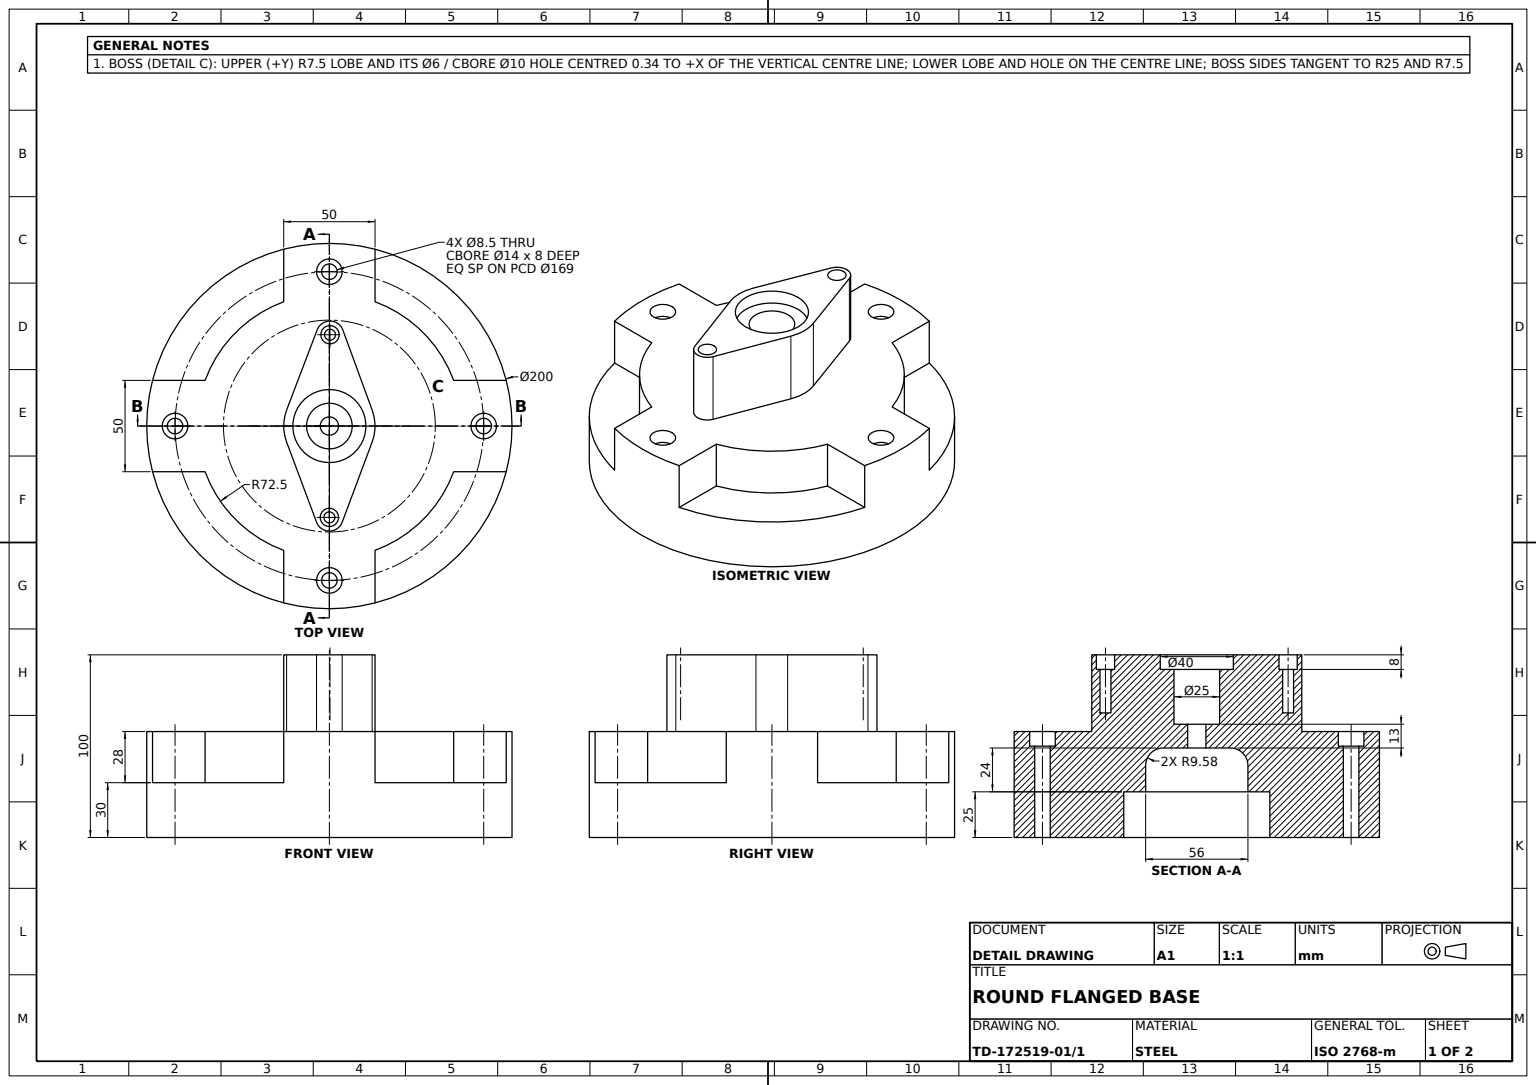
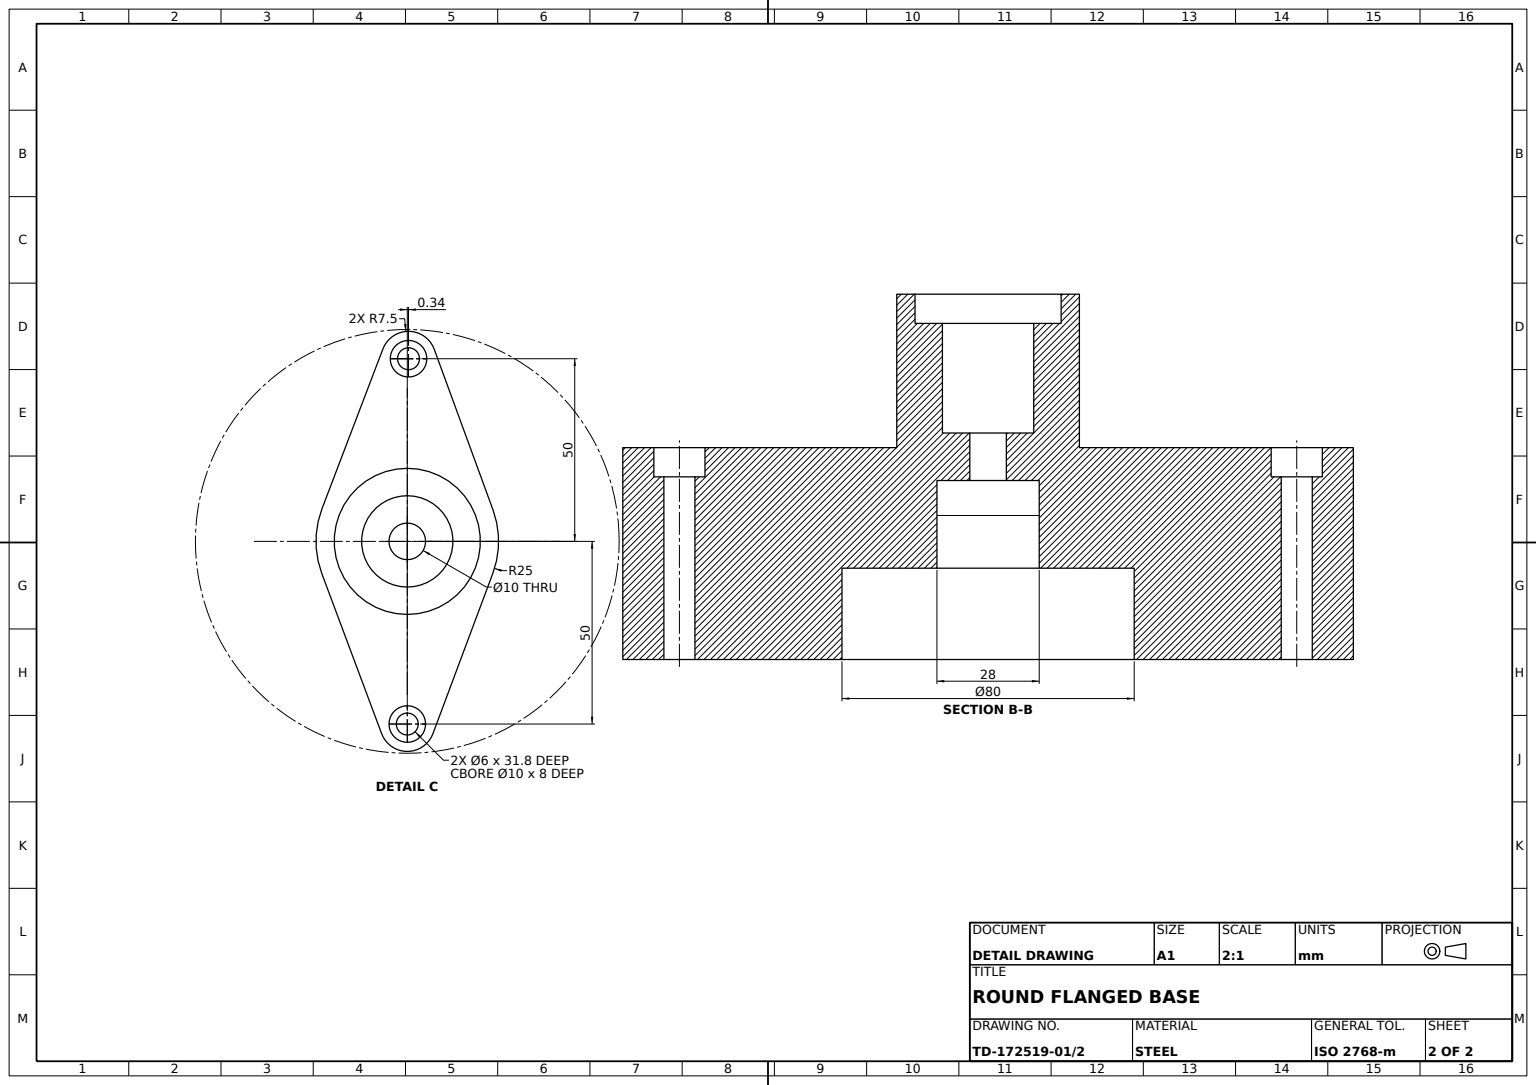
solid
v1 (0,68.2,53)
v2 (0,68.2,47)
e1 v1 v2 CIRCLE(AX(P(0,68.2,50),D(0,1,0),D(0,0,1)),3)
e2 v2 v1 CIRCLE(AX(P(0,68.2,50),D(0,1,0),D(0,0,1)),3)
face PLANE(AX(P(0,68.2,50),D(0,1,0),D(0,0,1))) [e1 e2]
v3 (0,58,-91.5)
v4 (0,58,-77.5)
e3 v3 v4 CIRCLE(AX(P(0,58,-84.5),D(0,1,0),D(0,0,1)),7)
e4 v4 v3 CIRCLE(AX(P(0,58,-84.5),D(0,1,0),D(0,0,1)),7)
v5 (25,58,68.053288)
v6 (68.053288,58,25)
e5 v5 v6 CIRCLE(AX(P(0,58,0),D(0,1,0),D(0,0,1)),72.5)
v7 (96.824584,58,25)
e6 v6 v7 LINE
v8 (96.824584,58,-25)
e7 v7 v8 CIRCLE(AX(P(0,58,0),D(0,1,0),D(0,0,1)),100)
v9 (68.053288,58,-25)
e8 v8 v9 LINE
v10 (25,58,-68.053288)
e9 v9 v10 CIRCLE(AX(P(0,58,0),D(0,1,0),D(0,0,1)),72.5)
v11 (25,58,-96.824584)
e10 v10 v11 LINE
v12 (0,58,-100)
e11 v11 v12 CIRCLE(AX(P(0,58,0),D(0,1,0),D(0,0,1)),100)
v13 (-25,58,-96.824584)
e12 v12 v13 CIRCLE(AX(P(0,58,0),D(0,1,0),D(0,0,1)),100)
v14 (-25,58,-68.053288)
e13 v13 v14 LINE
v15 (-68.053288,58,-25)
e14 v14 v15 CIRCLE(AX(P(0,58,0),D(0,1,0),D(0,0,1)),72.5)
v16 (-96.824584,58,-25)
e15 v15 v16 LINE
v17 (-96.824584,58,25)
e16 v16 v17 CIRCLE(AX(P(0,58,0),D(0,1,0),D(0,0,1)),100)
v18 (-68.053288,58,25)
e17 v17 v18 LINE
v19 (-25,58,68.053288)
e18 v18 v19 CIRCLE(AX(P(0,58,0),D(0,1,0),D(0,0,1)),72.5)
v20 (-25,58,96.824584)
e19 v19 v20 LINE
v21 (0,58,100)
e20 v20 v21 CIRCLE(AX(P(0,58,0),D(0,1,0),D(0,0,1)),100)
v22 (25,58,96.824584)
e21 v21 v22 CIRCLE(AX(P(0,58,0),D(0,1,0),D(0,0,1)),100)
e22 v22 v5 LINE
v23 (84.5,58,-7)
v24 (84.5,58,7)
e23 v23 v24 CIRCLE(AX(P(84.5,58,0),D(0,1,0),D(0,0,1)),7)
e24 v24 v23 CIRCLE(AX(P(84.5,58,0),D(0,1,0),D(0,0,1)),7)
v25 (0,58,77.5)
v26 (0,58,91.5)
e25 v25 v26 CIRCLE(AX(P(0,58,84.5),D(0,1,0),D(0,0,1)),7)
e26 v26 v25 CIRCLE(AX(P(0,58,84.5),D(0,1,0),D(0,0,1)),7)
v27 (7.025623,58,52.625)
v28 (23.418742,58,8.75)
e27 v27 v28 LINE
v29 (-7.025623,58,52.625)
e28 v29 v27 CIRCLE(AX(P(0,58,50),D(0,1,0),D(0,0,1)),7.5)
v30 (-23.418742,58,8.75)
e29 v30 v29 LINE
v31 (-23.359174,58,-8.907806)
e30 v31 v30 CIRCLE(AX(P(0,58,0),D(0,1,0),D(0,0,1)),25)
v32 (-6.670405,58,-52.671204)
e31 v32 v31 LINE
v33 (0.337347,58,-57.498862)
e32 v33 v32 CIRCLE(AX(P(0.337347,58,-49.998862),D(0,1,0),D(0,0,1)),7.5)
v34 (7.380521,58,-52.576401)
e33 v34 v33 CIRCLE(AX(P(0.337347,58,-49.998862),D(0,1,0),D(0,0,1)),7.5)
v35 (23.477245,58,-8.591796)
e34 v35 v34 LINE
e35 v28 v35 CIRCLE(AX(P(0,58,0),D(0,1,0),D(0,0,1)),25)
v36 (-84.5,58,7)
v37 (-84.5,58,-7)
e36 v36 v37 CIRCLE(AX(P(-84.5,58,0),D(0,1,0),D(0,0,1)),7)
e37 v37 v36 CIRCLE(AX(P(-84.5,58,0),D(0,1,0),D(0,0,1)),7)
face PLANE(AX(P(0,58,0),D(0,1,0),D(0,0,1))) [-e3 -e4] [e5 e6 e7 e8 e9 e10 e11 e12 e13 e14 e15 e16 e17 e18 e19 e20 e21 e22] [-e23 -e24] [-e25 -e26] [-e27 -e28 -e29 -e30 -e31 -e32 -e33 -e34 -e35] [-e36 -e37]
v38 (23.477245,100,-8.591796)
e38 v38 v35 LINE
v39 (23.418742,100,8.75)
e39 v39 v38 CIRCLE(AX(P(0,100,0),D(0,1,0),D(0,0,1)),25)
e40 v39 v28 LINE
face CYL(AX(P(0,100,0),D(0,-1,0),D(0,0,-1)),25) [-e38 -e39 e40 e35]
v40 (0,0,80.25)
v41 (0,0,88.75)
e41 v40 v41 CIRCLE(AX(P(0,0,84.5),D(0,1,0),D(0,0,1)),4.25)
e42 v41 v40 CIRCLE(AX(P(0,0,84.5),D(0,1,0),D(0,0,1)),4.25)
v42 (0,0,-80.25)
v43 (0,0,-88.75)
e43 v42 v43 CIRCLE(AX(P(0,0,-84.5),D(0,1,0),D(0,0,1)),4.25)
e44 v43 v42 CIRCLE(AX(P(0,0,-84.5),D(0,1,0),D(0,0,1)),4.25)
v44 (0,0,-100)
v45 (0,0,100)
e45 v44 v45 CIRCLE(AX(P(0,0,0),D(0,1,0),D(0,0,1)),100)
e46 v45 v44 CIRCLE(AX(P(0,0,0),D(0,1,0),D(0,0,1)),100)
v46 (-84.5,0,4.25)
v47 (-84.5,0,-4.25)
e47 v46 v47 CIRCLE(AX(P(-84.5,0,0),D(0,1,0),D(0,0,1)),4.25)
e48 v47 v46 CIRCLE(AX(P(-84.5,0,0),D(0,1,0),D(0,0,1)),4.25)
v48 (84.5,0,4.25)
v49 (84.5,0,-4.25)
e49 v48 v49 CIRCLE(AX(P(84.5,0,0),D(0,1,0),D(0,0,1)),4.25)
e50 v49 v48 CIRCLE(AX(P(84.5,0,0),D(0,1,0),D(0,0,1)),4.25)
v50 (0,0,-40)
v51 (0,0,40)
e51 v50 v51 CIRCLE(AX(P(0,0,0),D(0,-1,0),D(0,0,-1)),40)
e52 v51 v50 CIRCLE(AX(P(0,0,0),D(0,-1,0),D(0,0,-1)),40)
face PLANE(AX(P(0,0,0),D(0,1,0),D(0,0,1))) rev [e41 e42] [e43 e44] [-e45 -e46] [e47 e48] [e49 e50] [-e51 -e52]
v52 (-84.5,50,7)
e53 v52 v36 LINE
v53 (-84.5,50,-7)
e54 v53 v37 LINE
e55 v52 v53 CIRCLE(AX(P(-84.5,50,0),D(0,1,0),D(0,0,1)),7)
face CYL(AX(P(-84.5,50,0),D(0,1,0),D(0,0,1)),7) rev [e53 e36 -e54 -e55]
v54 (0.337347,100,-44.998862)
v55 (0.337347,100,-54.998862)
e56 v54 v55 CIRCLE(AX(P(0.337347,100,-49.998862),D(0,1,0),D(0,0,1)),5)
v56 (0.337347,92,-54.998862)
e57 v56 v55 LINE
v57 (0.337347,92,-44.998862)
e58 v57 v56 CIRCLE(AX(P(0.337347,92,-49.998862),D(0,1,0),D(0,0,1)),5)
e59 v57 v54 LINE
face CYL(AX(P(0.337347,92,-49.998862),D(0,1,0),D(0,0,1)),5) rev [e56 -e57 -e58 e59]
v58 (0.337347,68.2,-52.998862)
v59 (0.337347,68.2,-46.998862)
e60 v58 v59 CIRCLE(AX(P(0.337347,68.2,-49.998862),D(0,1,0),D(0,0,1)),3)
e61 v59 v58 CIRCLE(AX(P(0.337347,68.2,-49.998862),D(0,1,0),D(0,0,1)),3)
face PLANE(AX(P(0.337347,68.2,-49.998862),D(0,1,0),D(0,0,1))) [e60 e61]
v60 (-96.824584,30,25)
v61 (-25,30,96.824584)
e62 v60 v61 CIRCLE(AX(P(0,30,0),D(0,1,0),D(0,0,1)),100)
v62 (-25,30,68.053288)
e63 v62 v61 LINE
v63 (-68.053288,30,25)
e64 v63 v62 CIRCLE(AX(P(0,30,0),D(0,1,0),D(0,0,1)),72.5)
e65 v60 v63 LINE
face PLANE(AX(P(0,30,0),D(0,1,0),D(0,0,1))) [e62 -e63 -e64 -e65]
v64 (-84.5,50,-4.25)
e66 v47 v64 LINE
v65 (-84.5,50,4.25)
e67 v64 v65 CIRCLE(AX(P(-84.5,50,0),D(0,1,0),D(0,0,1)),4.25)
e68 v46 v65 LINE
face CYL(AX(P(-84.5,0,0),D(0,1,0),D(0,0,1)),4.25) rev [-e48 e66 e67 -e68]
v66 (0,92,-20)
v67 (0,92,20)
e69 v66 v67 CIRCLE(AX(P(0,92,0),D(0,1,0),D(0,0,1)),20)
v68 (0,100,-20)
e70 v66 v68 LINE
v69 (0,100,20)
e71 v68 v69 CIRCLE(AX(P(0,100,0),D(0,1,0),D(0,0,1)),20)
e72 v67 v69 LINE
face CYL(AX(P(0,92,0),D(0,1,0),D(0,0,1)),20) rev [-e69 e70 e71 -e72]
v70 (7.380521,100,-52.576401)
e73 v70 v34 LINE
e74 v38 v70 LINE
face PLANE(AX(P(7.380521,100,-52.576401),D(-0.939089811,0,0.343671832),D(0.343671832,0,0.939089811))) rev [e34 -e73 -e74 e38]
v71 (25,30,68.053288)
e75 v5 v71 LINE
v72 (25,30,96.824584)
e76 v22 v72 LINE
e77 v72 v71 LINE
face PLANE(AX(P(25,58,68.053288),D(-1,0,0),D(0,0,1))) rev [-e75 -e22 e76 e77]
e78 v55 v54 CIRCLE(AX(P(0.337347,100,-49.998862),D(0,1,0),D(0,0,1)),5)
e79 v56 v57 CIRCLE(AX(P(0.337347,92,-49.998862),D(0,1,0),D(0,0,1)),5)
face CYL(AX(P(0.337347,92,-49.998862),D(0,1,0),D(0,0,1)),5) rev [e57 e78 -e59 -e79]
v73 (96.824584,30,-25)
v74 (68.053288,30,-25)
e80 v73 v74 LINE
e81 v9 v74 LINE
e82 v8 v73 LINE
face PLANE(AX(P(68.053288,58,-25),D(0,0,1),D(1,0,0))) rev [e80 -e81 -e8 e82]
v75 (-68.053288,30,-25)
v76 (-96.824584,30,-25)
e83 v75 v76 LINE
e84 v16 v76 LINE
e85 v15 v75 LINE
face PLANE(AX(P(-68.053288,58,-25),D(0,0,1),D(1,0,0))) rev [e83 -e84 -e15 e85]
v77 (84.5,50,7)
e86 v77 v24 LINE
v78 (84.5,50,-7)
e87 v78 v77 CIRCLE(AX(P(84.5,50,0),D(0,1,0),D(0,0,1)),7)
e88 v78 v23 LINE
face CYL(AX(P(84.5,50,0),D(0,1,0),D(0,0,1)),7) rev [-e86 -e87 e88 e23]
v79 (0,50,88.75)
e89 v41 v79 LINE
v80 (0,50,80.25)
e90 v79 v80 CIRCLE(AX(P(0,50,84.5),D(0,1,0),D(0,0,1)),4.25)
e91 v40 v80 LINE
face CYL(AX(P(0,0,84.5),D(0,1,0),D(0,0,1)),4.25) rev [-e42 e89 e90 -e91]
v81 (7.025623,100,52.625)
e92 v81 v39 LINE
e93 v81 v27 LINE
face PLANE(AX(P(7.025623,100,52.625),D(-0.9367497,0,-0.35),D(-0.35,0,0.9367497))) rev [e27 -e40 -e92 e93]
v82 (-23.359174,100,-8.907806)
e94 v82 v31 LINE
v83 (-6.670405,100,-52.671204)
e95 v83 v82 LINE
e96 v83 v32 LINE
face PLANE(AX(P(-6.670405,100,-52.671204),D(0.934366946,0,0.356312236),D(0.356312236,0,-0.934366946))) rev [-e94 -e95 e96 e31]
v84 (-23.418742,100,8.75)
v85 (-7.025623,100,52.625)
e97 v84 v85 LINE
e98 v84 v30 LINE
e99 v85 v29 LINE
face PLANE(AX(P(-7.025623,100,52.625),D(0.9367497,0,-0.35),D(-0.35,0,-0.9367497))) rev [-e97 e98 e29 -e99]
v86 (14,39.42,-28)
v87 (14,49,-18.42)
e100 v86 v87 CIRCLE(AX(P(14,39.42,-18.42),D(1,0,0),D(0,0,-1)),9.58)
v88 (-14,49,-18.42)
e101 v88 v87 LINE
v89 (-14,39.42,-28)
e102 v89 v88 CIRCLE(AX(P(-14,39.42,-18.42),D(1,0,0),D(0,0,-1)),9.58)
e103 v89 v86 LINE
face CYL(AX(P(-14,39.42,-18.42),D(1,0,0),D(0,0,-1)),9.58) rev [e100 -e101 -e102 e103]
v90 (0.337347,100,-57.498862)
e104 v90 v33 LINE
e105 v70 v90 CIRCLE(AX(P(0.337347,100,-49.998862),D(0,1,0),D(0,0,1)),7.5)
face CYL(AX(P(0.337347,100,-49.998862),D(0,-1,0),D(0,0,-1)),7.5) [e33 -e104 -e105 e73]
e106 v80 v79 CIRCLE(AX(P(0,50,84.5),D(0,1,0),D(0,0,1)),4.25)
v91 (0,50,77.5)
v92 (0,50,91.5)
e107 v91 v92 CIRCLE(AX(P(0,50,84.5),D(0,1,0),D(0,0,1)),7)
e108 v92 v91 CIRCLE(AX(P(0,50,84.5),D(0,1,0),D(0,0,1)),7)
face PLANE(AX(P(0,50,84.5),D(0,1,0),D(0,0,1))) [-e106 -e90] [e107 e108]
v93 (0,25,-40)
e109 v93 v50 LINE
v94 (0,25,40)
e110 v94 v93 CIRCLE(AX(P(0,25,0),D(0,-1,0),D(0,0,-1)),40)
e111 v94 v51 LINE
face CYL(AX(P(0,25,0),D(0,-1,0),D(0,0,-1)),40) rev [e52 -e109 -e110 e111]
v95 (25,30,-96.824584)
e112 v11 v95 LINE
v96 (25,30,-68.053288)
e113 v10 v96 LINE
e114 v96 v95 LINE
face PLANE(AX(P(25,58,-68.053288),D(-1,0,0),D(0,0,1))) rev [-e112 -e10 e113 e114]
v97 (-14,49,18.42)
v98 (-14,39.42,28)
e115 v97 v98 CIRCLE(AX(P(-14,39.42,18.42),D(1,0,0),D(0,0,-1)),9.58)
v99 (-14,25,28)
e116 v98 v99 LINE
v100 (-14,25,-28)
e117 v99 v100 LINE
e118 v100 v89 LINE
e119 v88 v97 LINE
face PLANE(AX(P(-14,39.42,18.42),D(1,0,0),D(0,0,-1))) [e115 e116 e117 e118 e102 e119]
v101 (14,39.42,28)
e120 v98 v101 LINE
v102 (14,25,28)
e121 v101 v102 LINE
e122 v99 v102 LINE
face PLANE(AX(P(-14,25,28),D(0,0,1),D(1,0,0))) rev [e120 e121 -e122 -e116]
v103 (0.337347,92,-52.998862)
v104 (0.337347,92,-46.998862)
e123 v103 v104 CIRCLE(AX(P(0.337347,92,-49.998862),D(0,1,0),D(0,0,1)),3)
e124 v104 v103 CIRCLE(AX(P(0.337347,92,-49.998862),D(0,1,0),D(0,0,1)),3)
face PLANE(AX(P(0.337347,92,-49.998862),D(0,1,0),D(0,0,1))) [e79 e58] [-e123 -e124]
e125 v67 v66 CIRCLE(AX(P(0,92,0),D(0,1,0),D(0,0,1)),20)
e126 v69 v68 CIRCLE(AX(P(0,100,0),D(0,1,0),D(0,0,1)),20)
face CYL(AX(P(0,92,0),D(0,1,0),D(0,0,1)),20) rev [-e70 -e125 e72 e126]
e127 v93 v94 CIRCLE(AX(P(0,25,0),D(0,-1,0),D(0,0,-1)),40)
v105 (14,25,-28)
e128 v102 v105 LINE
e129 v100 v105 LINE
face PLANE(AX(P(0,25,0),D(0,-1,0),D(0,0,-1))) [e110 e127] [e122 e128 -e129 -e117]
v106 (0,50,-88.75)
v107 (0,50,-80.25)
e130 v106 v107 CIRCLE(AX(P(0,50,-84.5),D(0,1,0),D(0,0,1)),4.25)
e131 v107 v106 CIRCLE(AX(P(0,50,-84.5),D(0,1,0),D(0,0,1)),4.25)
v108 (0,50,-77.5)
v109 (0,50,-91.5)
e132 v108 v109 CIRCLE(AX(P(0,50,-84.5),D(0,1,0),D(0,0,1)),7)
e133 v109 v108 CIRCLE(AX(P(0,50,-84.5),D(0,1,0),D(0,0,1)),7)
face PLANE(AX(P(0,50,-84.5),D(0,1,0),D(0,0,1))) [-e130 -e131] [e132 e133]
e134 v59 v104 LINE
e135 v58 v103 LINE
face CYL(AX(P(0.337347,68.2,-49.998862),D(0,1,0),D(0,0,1)),3) rev [-e61 e134 e124 -e135]
v110 (0,92,53)
e136 v1 v110 LINE
v111 (0,92,47)
e137 v110 v111 CIRCLE(AX(P(0,92,50),D(0,1,0),D(0,0,1)),3)
e138 v2 v111 LINE
face CYL(AX(P(0,68.2,50),D(0,1,0),D(0,0,1)),3) rev [e136 e137 -e138 -e1]
e139 v82 v84 CIRCLE(AX(P(0,100,0),D(0,1,0),D(0,0,1)),25)
face CYL(AX(P(0,100,0),D(0,-1,0),D(0,0,-1)),25) [e30 -e98 -e139 e94]
v112 (-25,30,-96.824584)
e140 v13 v112 LINE
v113 (-25,30,-68.053288)
e141 v112 v113 LINE
e142 v14 v113 LINE
face PLANE(AX(P(-25,58,-68.053288),D(1,0,0),D(0,0,-1))) rev [-e13 e140 e141 -e142]
e143 v112 v76 CIRCLE(AX(P(0,30,0),D(0,1,0),D(0,0,1)),100)
e144 v113 v75 CIRCLE(AX(P(0,30,0),D(0,1,0),D(0,0,1)),72.5)
face PLANE(AX(P(0,30,0),D(0,1,0),D(0,0,1))) [-e141 e143 -e83 -e144]
face CYL(AX(P(0,0,84.5),D(0,1,0),D(0,0,1)),4.25) rev [-e89 -e41 e91 e106]
e145 v92 v26 LINE
e146 v91 v25 LINE
face CYL(AX(P(0,50,84.5),D(0,1,0),D(0,0,1)),7) rev [e145 e26 -e146 -e108]
face CYL(AX(P(0,25,0),D(0,-1,0),D(0,0,-1)),40) rev [e51 -e111 -e127 e109]
e147 v65 v64 CIRCLE(AX(P(-84.5,50,0),D(0,1,0),D(0,0,1)),4.25)
face CYL(AX(P(-84.5,0,0),D(0,1,0),D(0,0,1)),4.25) rev [e68 e147 -e66 -e47]
e148 v73 v95 CIRCLE(AX(P(0,30,0),D(0,1,0),D(0,0,1)),100)
e149 v74 v96 CIRCLE(AX(P(0,30,0),D(0,1,0),D(0,0,1)),72.5)
face PLANE(AX(P(0,30,0),D(0,1,0),D(0,0,1))) [e148 -e114 -e149 -e80]
e150 v53 v52 CIRCLE(AX(P(-84.5,50,0),D(0,1,0),D(0,0,1)),7)
face CYL(AX(P(-84.5,50,0),D(0,1,0),D(0,0,1)),7) rev [e54 e37 -e53 -e150]
face CYL(AX(P(0.337347,68.2,-49.998862),D(0,1,0),D(0,0,1)),3) rev [e135 e123 -e134 -e60]
v114 (68.053288,30,25)
e151 v71 v114 CIRCLE(AX(P(0,30,0),D(0,1,0),D(0,0,1)),72.5)
e152 v6 v114 LINE
face CYL(AX(P(0,58,0),D(0,-1,0),D(0,0,-1)),72.5) [e75 e151 -e152 -e5]
e153 v77 v78 CIRCLE(AX(P(84.5,50,0),D(0,1,0),D(0,0,1)),7)
v115 (84.5,50,4.25)
v116 (84.5,50,-4.25)
e154 v115 v116 CIRCLE(AX(P(84.5,50,0),D(0,1,0),D(0,0,1)),4.25)
e155 v116 v115 CIRCLE(AX(P(84.5,50,0),D(0,1,0),D(0,0,1)),4.25)
face PLANE(AX(P(84.5,50,0),D(0,1,0),D(0,0,1))) [e153 e87] [-e154 -e155]
face PLANE(AX(P(-84.5,50,0),D(0,1,0),D(0,0,1))) [-e67 -e147] [e150 e55]
e156 v49 v116 LINE
e157 v48 v115 LINE
face CYL(AX(P(84.5,0,0),D(0,1,0),D(0,0,1)),4.25) rev [-e50 e156 e155 -e157]
e158 v19 v62 LINE
e159 v18 v63 LINE
face CYL(AX(P(0,58,0),D(0,-1,0),D(0,0,-1)),72.5) [-e158 -e18 e159 e64]
v117 (0,49,5)
v118 (0,62,5)
e160 v117 v118 LINE
v119 (0,49,-5)
e161 v117 v119 CIRCLE(AX(P(0,49,0),D(0,-1,0),D(0,0,1)),5)
v120 (0,62,-5)
e162 v119 v120 LINE
e163 v120 v118 CIRCLE(AX(P(0,62,0),D(0,1,0),D(0,0,1)),5)
face CYL(AX(P(0,49,0),D(0,1,0),D(0,0,1)),5) rev [-e160 e161 e162 e163]
v121 (14,49,18.42)
e164 v97 v121 LINE
e165 v121 v101 CIRCLE(AX(P(14,39.42,18.42),D(1,0,0),D(0,0,-1)),9.58)
face CYL(AX(P(-14,39.42,18.42),D(1,0,0),D(0,0,-1)),9.58) rev [e164 e165 -e120 -e115]
v122 (0,62,-12.5)
v123 (0,62,12.5)
e166 v122 v123 CIRCLE(AX(P(0,62,0),D(0,1,0),D(0,0,1)),12.5)
e167 v123 v122 CIRCLE(AX(P(0,62,0),D(0,1,0),D(0,0,1)),12.5)
e168 v118 v120 CIRCLE(AX(P(0,62,0),D(0,1,0),D(0,0,1)),5)
face PLANE(AX(P(0,62,0),D(0,1,0),D(0,0,1))) [e166 e167] [-e168 -e163]
face CYL(AX(P(84.5,0,0),D(0,1,0),D(0,0,1)),4.25) rev [-e49 e157 e154 -e156]
face CYL(AX(P(0,50,84.5),D(0,1,0),D(0,0,1)),7) rev [e25 -e145 -e107 e146]
e169 v85 v81 CIRCLE(AX(P(0,100,50),D(0,1,0),D(0,0,1)),7.5)
e170 v90 v83 CIRCLE(AX(P(0.337347,100,-49.998862),D(0,1,0),D(0,0,1)),7.5)
v124 (0,100,45)
v125 (0,100,55)
e171 v124 v125 CIRCLE(AX(P(0,100,50),D(0,1,0),D(0,0,1)),5)
e172 v125 v124 CIRCLE(AX(P(0,100,50),D(0,1,0),D(0,0,1)),5)
face PLANE(AX(P(0.337347,100,-49.998862),D(0,1,0),D(0,0,1))) [-e78 -e56] [e95 e139 e97 e169 e92 e39 e74 e105 e170] [-e171 -e172] [-e126 -e71]
face CYL(AX(P(0.337347,100,-49.998862),D(0,-1,0),D(0,0,-1)),7.5) [e104 e32 -e96 -e170]
e173 v17 v60 LINE
e174 v12 v44 LINE
e175 v21 v45 LINE
e176 v20 v61 LINE
face CYL(AX(P(0,30,0),D(0,-1,0),D(0,0,-1)),100) [-e173 -e16 e84 -e143 -e140 -e12 e174 e45 -e175 -e20 e176 -e62]
e177 v111 v110 CIRCLE(AX(P(0,92,50),D(0,1,0),D(0,0,1)),3)
face CYL(AX(P(0,68.2,50),D(0,1,0),D(0,0,1)),3) rev [e177 -e136 -e2 e138]
e178 v119 v117 CIRCLE(AX(P(0,49,0),D(0,-1,0),D(0,0,1)),5)
face CYL(AX(P(0,49,0),D(0,1,0),D(0,0,1)),5) rev [e160 e168 -e162 e178]
v126 (0,92,55)
e179 v126 v125 LINE
v127 (0,92,45)
e180 v127 v126 CIRCLE(AX(P(0,92,50),D(0,1,0),D(0,0,1)),5)
e181 v127 v124 LINE
face CYL(AX(P(0,92,50),D(0,1,0),D(0,0,1)),5) rev [e171 -e179 -e180 e181]
face CYL(AX(P(0,58,0),D(0,-1,0),D(0,0,-1)),72.5) [e81 e149 -e113 -e9]
e182 v105 v86 LINE
face PLANE(AX(P(-14,25,-28),D(0,0,-1),D(-1,0,0))) rev [e182 -e103 -e118 e129]
v128 (96.824584,30,25)
e183 v7 v128 LINE
e184 v114 v128 LINE
face PLANE(AX(P(68.053288,58,25),D(0,0,-1),D(-1,0,0))) rev [-e183 -e6 e152 e184]
face PLANE(AX(P(-68.053288,58,25),D(0,0,-1),D(-1,0,0))) rev [e65 -e159 -e17 e173]
e185 v72 v128 CIRCLE(AX(P(0,30,0),D(0,1,0),D(0,0,1)),100)
face CYL(AX(P(0,30,0),D(0,-1,0),D(0,0,-1)),100) [-e148 -e82 -e7 e183 -e185 -e76 -e21 e175 e46 -e174 -e11 e112]
e186 v87 v121 LINE
face PLANE(AX(P(-14,49,18.42),D(0,1,0),D(0,0,1))) rev [-e178 -e161] [e101 e186 -e164 -e119]
e187 v42 v107 LINE
e188 v43 v106 LINE
face CYL(AX(P(0,0,-84.5),D(0,1,0),D(0,0,1)),4.25) rev [-e187 -e44 e188 e130]
v129 (0,92,12.5)
e189 v123 v129 LINE
v130 (0,92,-12.5)
e190 v129 v130 CIRCLE(AX(P(0,92,0),D(0,1,0),D(0,0,1)),12.5)
e191 v122 v130 LINE
face CYL(AX(P(0,62,0),D(0,1,0),D(0,0,1)),12.5) rev [e189 e190 -e191 -e167]
e192 v126 v127 CIRCLE(AX(P(0,92,50),D(0,1,0),D(0,0,1)),5)
face PLANE(AX(P(0,92,50),D(0,1,0),D(0,0,1))) [e192 e180] [-e137 -e177]
face CYL(AX(P(0,58,0),D(0,-1,0),D(0,0,-1)),72.5) [e144 -e85 -e14 e142]
face PLANE(AX(P(-25,58,68.053288),D(1,0,0),D(0,0,-1))) rev [-e19 e158 e63 -e176]
face CYL(AX(P(84.5,50,0),D(0,1,0),D(0,0,1)),7) rev [e86 e24 -e88 -e153]
e193 v109 v3 LINE
e194 v108 v4 LINE
face CYL(AX(P(0,50,-84.5),D(0,1,0),D(0,0,1)),7) rev [e193 e3 -e194 -e133]
face CYL(AX(P(0,100,50),D(0,-1,0),D(0,0,-1)),7.5) [-e93 -e169 e99 e28]
face CYL(AX(P(0,50,-84.5),D(0,1,0),D(0,0,1)),7) rev [-e132 e194 e4 -e193]
face PLANE(AX(P(0,30,0),D(0,1,0),D(0,0,1))) [-e151 -e77 e185 -e184]
e195 v130 v129 CIRCLE(AX(P(0,92,0),D(0,1,0),D(0,0,1)),12.5)
face CYL(AX(P(0,62,0),D(0,1,0),D(0,0,1)),12.5) rev [-e189 -e166 e191 e195]
face PLANE(AX(P(14,39.42,18.42),D(1,0,0),D(0,0,-1))) rev [-e100 -e182 -e128 -e121 -e165 -e186]
face PLANE(AX(P(0,92,0),D(0,1,0),D(0,0,1))) [-e195 -e190] [e69 e125]
face CYL(AX(P(0,92,50),D(0,1,0),D(0,0,1)),5) rev [-e181 -e192 e179 e172]
face CYL(AX(P(0,0,-84.5),D(0,1,0),D(0,0,1)),4.25) rev [e187 e131 -e188 -e43]
